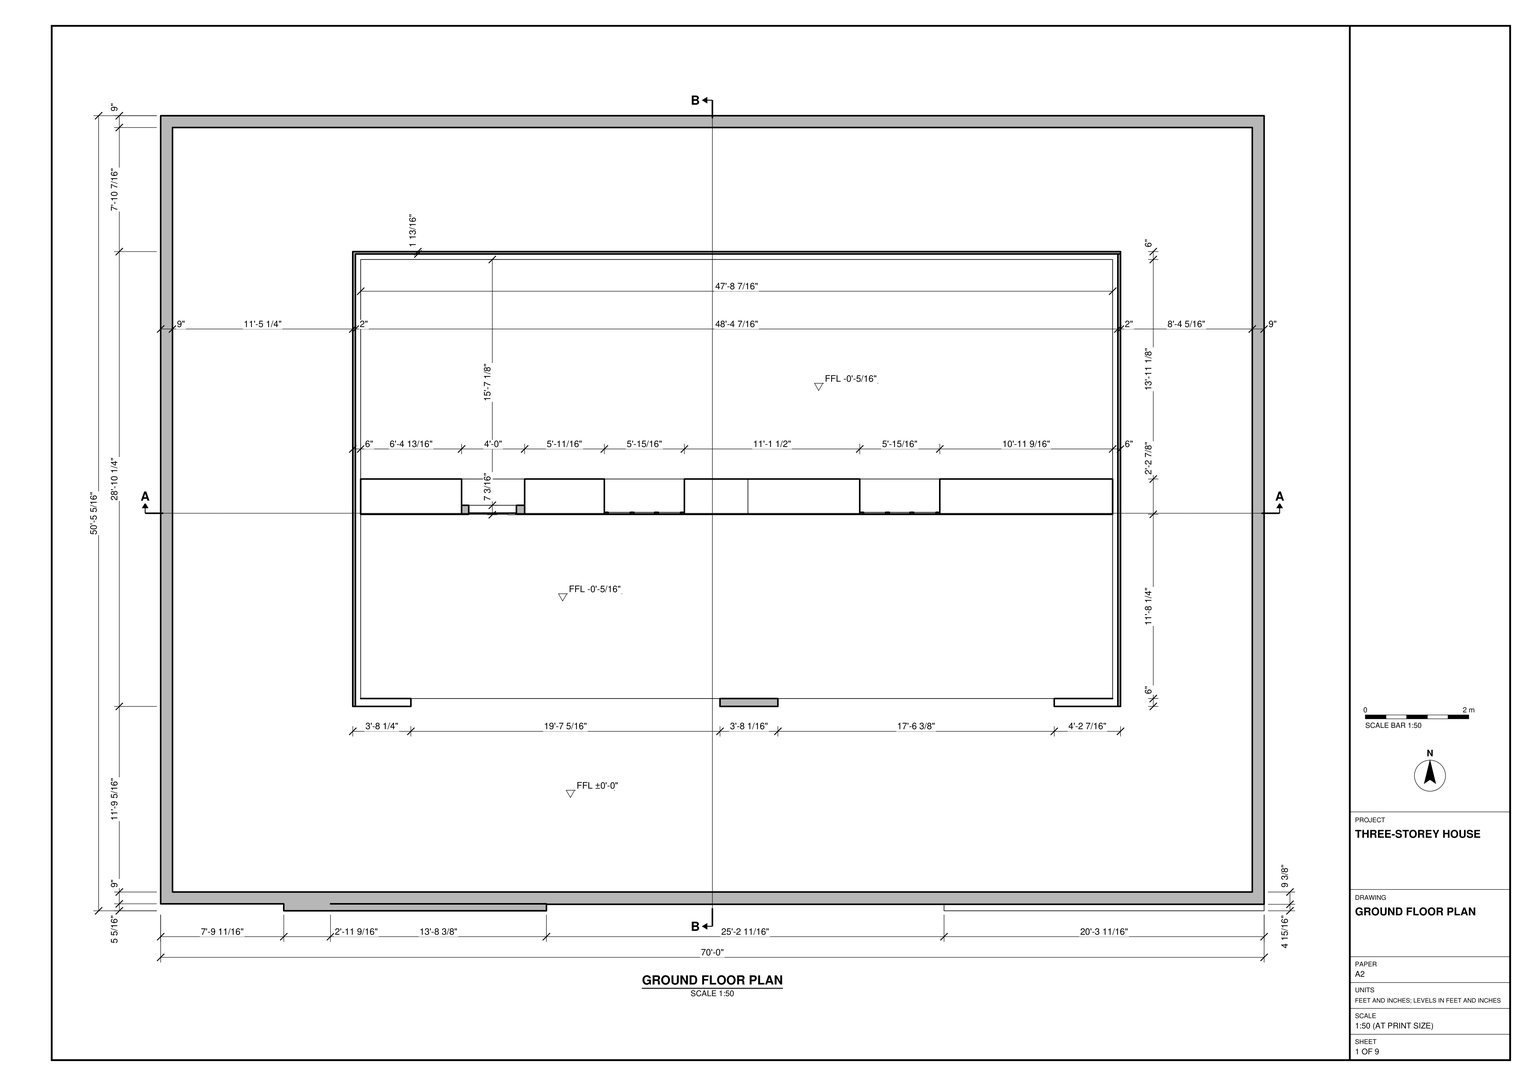
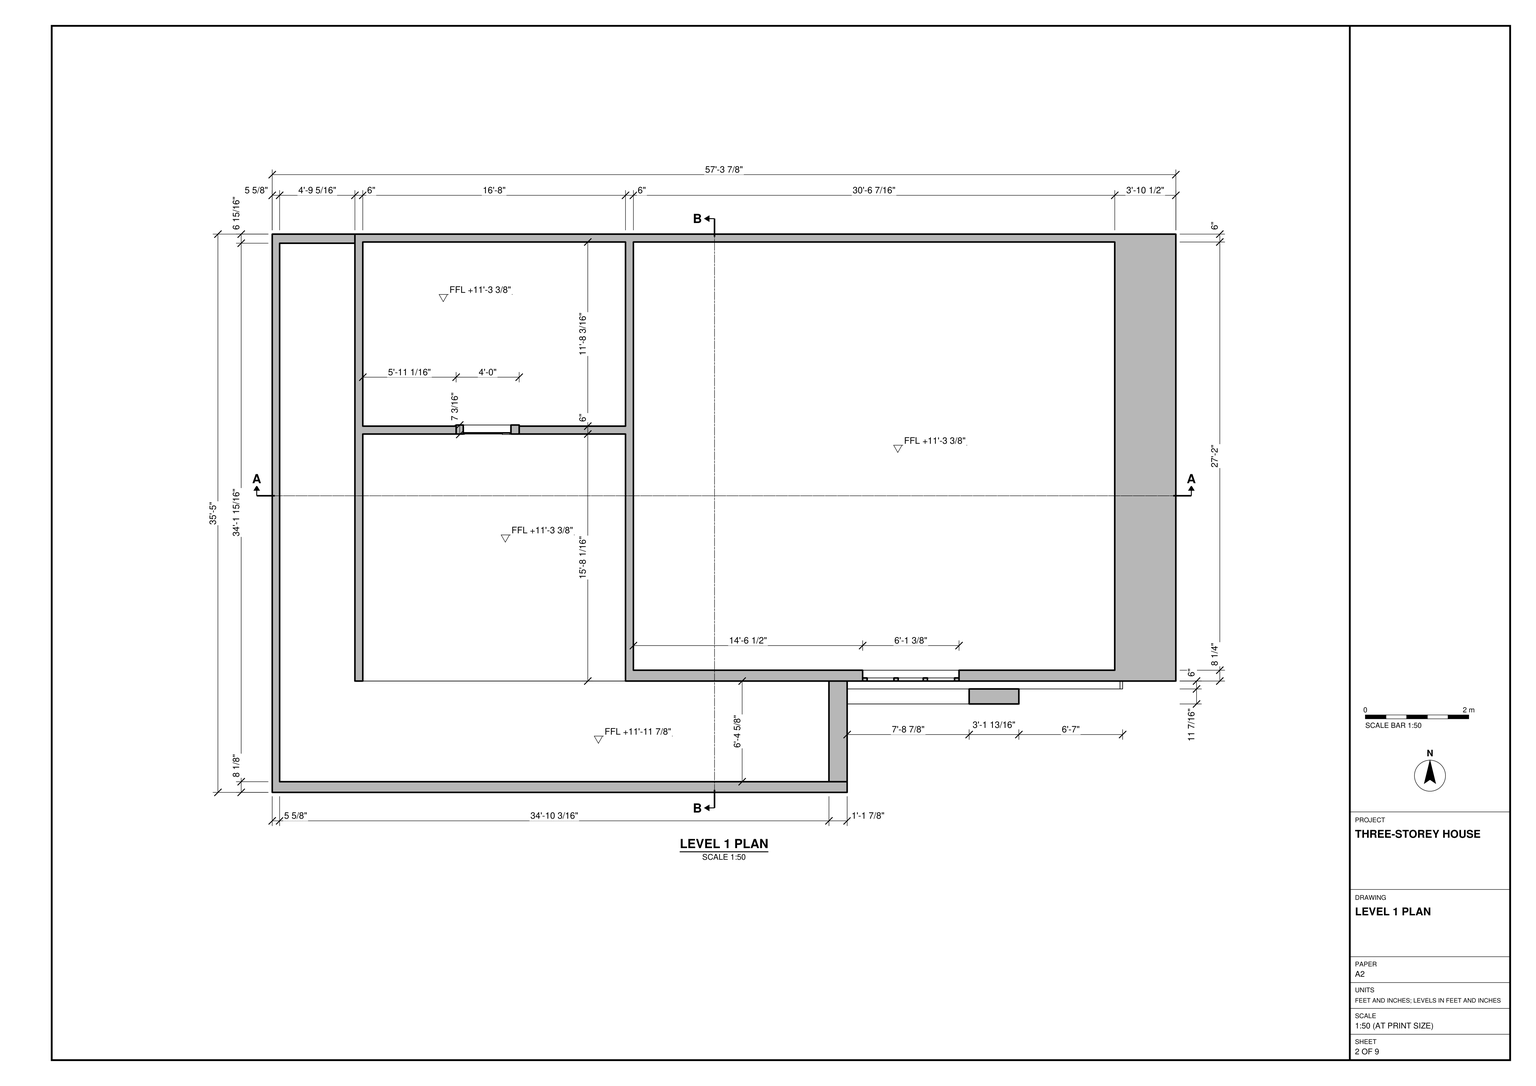
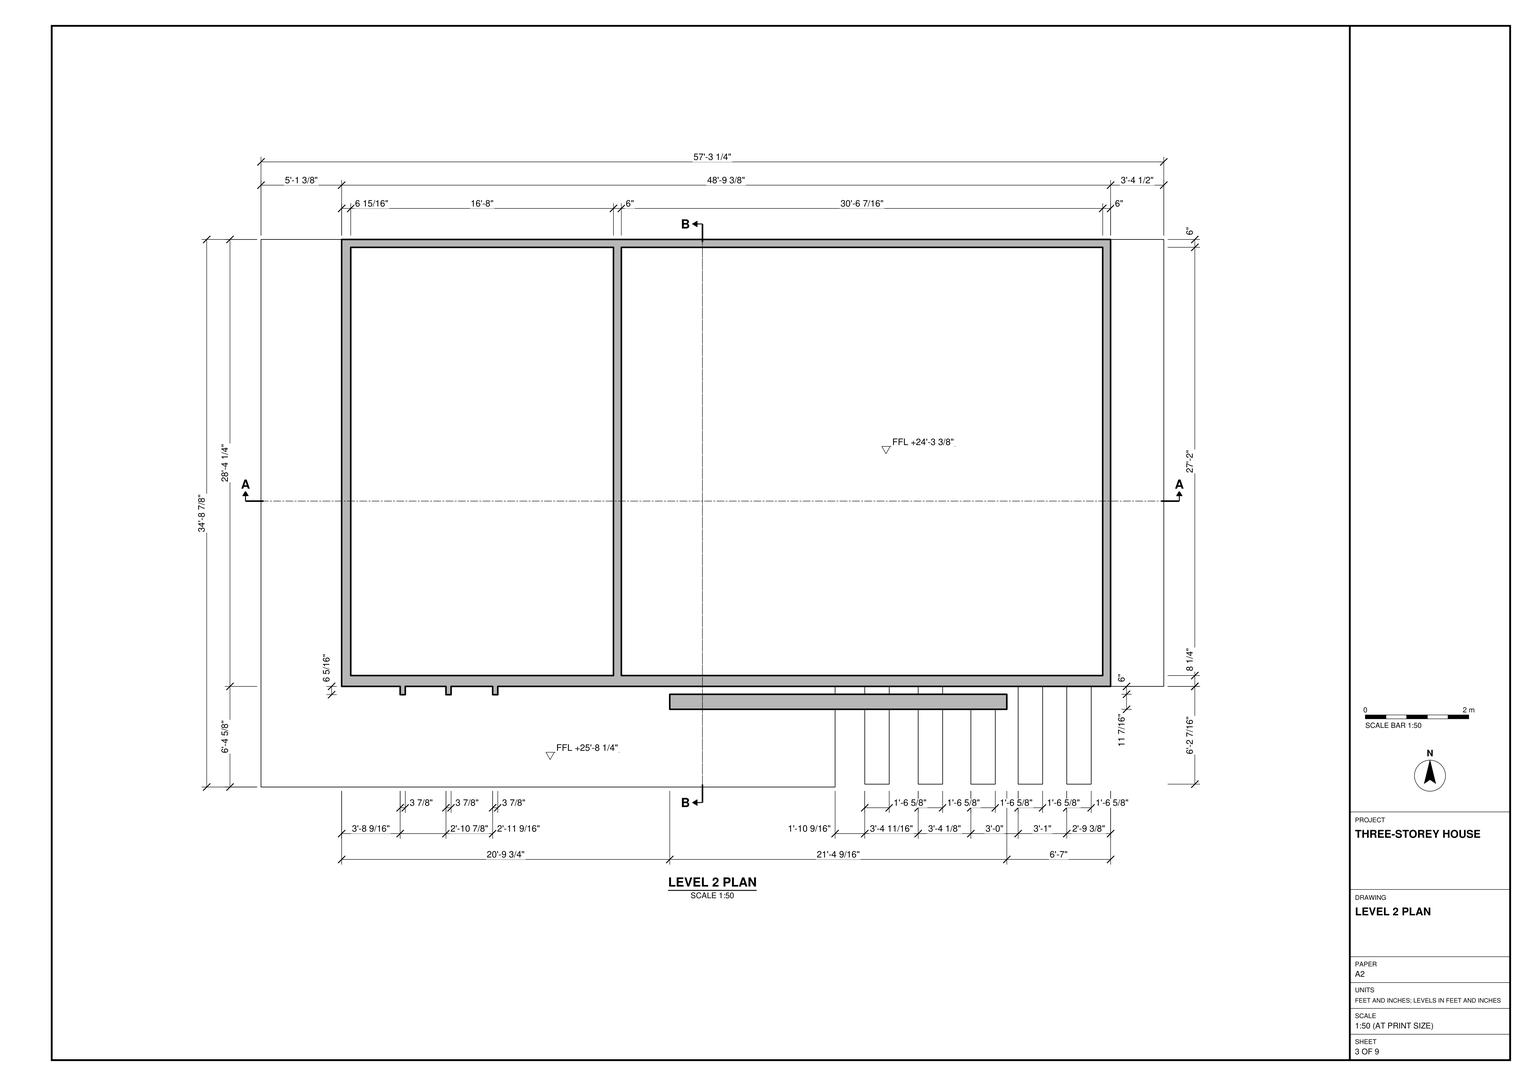
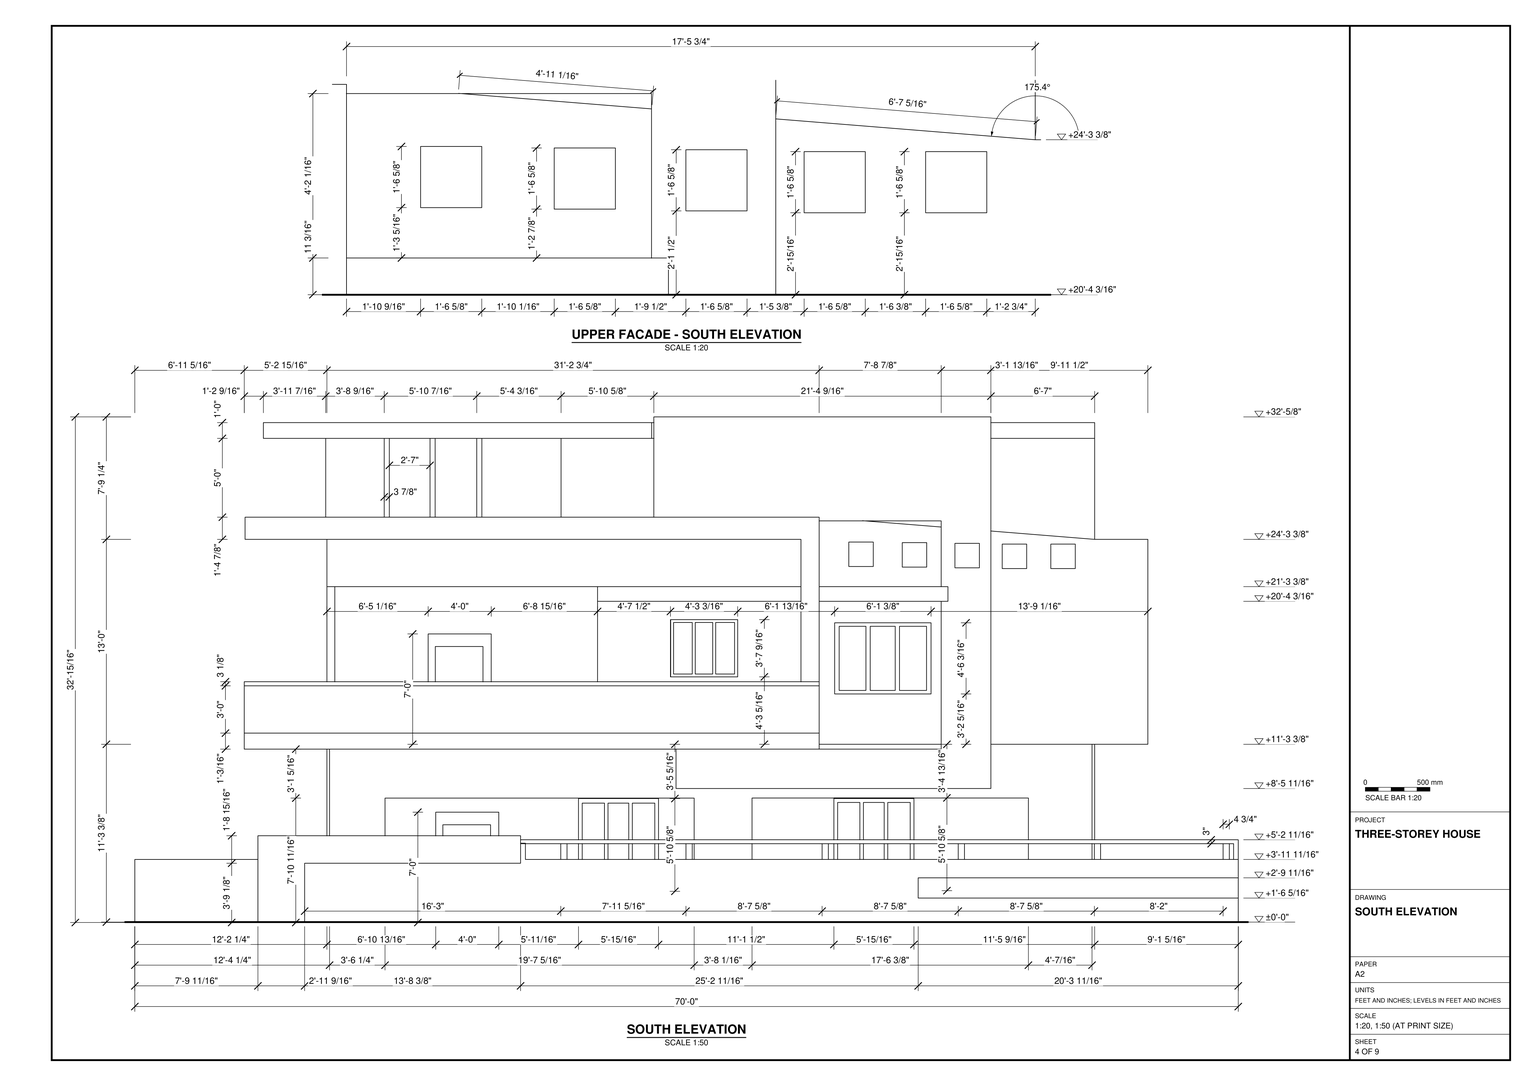
Build the house and its rectangular site perimeter in SketchUp using task_files/diagram_01.pdf. Work in feet and inches. The overall model is 70'-0" along X, 50'-5 5/16" along Y and 32'-15/16" high. Set the ground datum at ±0'-0", Level 1 at +11'-3 3/8" and Level 2 at +24'-3 3/8".

Set out the ground-floor footprint inside the perimeter, preserving the different setbacks on each side. Form the two wide openings along the front edge and the wall with openings between the front and rear spaces. At Level 1, lay out the smaller spaces on the left and the larger space on the right. Follow the stepped slab edge around the left side and across the front-left portion. At Level 2, align the lengthwise dividing wall with the division below. Model the roof edges, parallel projections at the front right and the member running across them.

Use the wall and slab thicknesses shown, and place door and window openings in the corresponding wall bays. Include stairs, built-in joinery and main furniture where shown. Keep shell elements such as walls, slabs and roof, and each furniture or joinery piece, in separate groups or components. Use components for repeated parts. Decor and loose items may be any suitable library components. Save one SketchUp model as output_files/three_storey_house_stepped_slabs_and_projecting_beams.skp.

# SketchUp Ruby script. Lengths in inches.
U = 1.inch
M = Sketchup.active_model
def pt(a) = Geom::Point3d.new(a.map { |v| v * U })
def face(e, loops, mat)
  f = e.add_face(loops[0].map { |a| pt(a) })
  loops[1..].each { |l| e.add_face(l.map { |a| pt(a) }).erase! }
  f.material = f.back_material = mat if mat
  f
end
# faces: each face lists its corners as indices into pts; further lists are holes
def faces(e, pts, list, mat = nil) = list.each { |f| face(e, (f[0].is_a?(Array) ? f : [f]).map { |l| l.map { |i| pts[i] } }, mat) }
# xy, xz, yz: faces in a plane at the given z, y or x. An outline is a flat list of corners, or four numbers for a rectangle; further outlines are holes
def ring(l) = l.size == 4 ? [[l[0], l[1]], [l[2], l[1]], [l[2], l[3]], [l[0], l[3]]] : l.each_slice(2).to_a
def flat(e, list, mat, &to3) = list.each { |f| face(e, (f[0].is_a?(Array) ? f : [f]).map { |l| ring(l).map { |u, v| to3.(u, v) } }, mat) }
def xy(e, z, list, mat = nil) = flat(e, list, mat) { |x, y| [x, y, z] }
def xz(e, y, list, mat = nil) = flat(e, list, mat) { |x, z| [x, y, z] }
def yz(e, x, list, mat = nil) = flat(e, list, mat) { |y, z| [x, y, z] }
def lines(e, pts, list) = list.each { |a, b| e.add_line(pt(pts[a]), pt(pts[b])) }
# prism: a flat outline (further loops are holes) pulled along v
def prism(e, loops, v, mat = nil)
  f = face(e, loops, mat); d = Geom::Vector3d.new(v.map { |x| x * U })
  f.pushpull(f.normal.samedirection?(d) ? d.length : -d.length)
end
def box(e, o, s, mat = nil) = prism(e, [[o, [o[0] + s[0], o[1], o[2]], [o[0] + s[0], o[1] + s[1], o[2]], [o[0], o[1] + s[1], o[2]]]], [0, 0, s[2]], mat)
def at(x, y, z, deg = 0) = Geom::Transformation.translation(pt([x, y, z])) * Geom::Transformation.rotation(ORIGIN, Z_AXIS, deg.degrees)
def axes(o, x, y, z) = Geom::Transformation.new([*x, 0, *y, 0, *z, 0, *pt(o).to_a, 1])
def part(name) = M.definitions.add(name)
# library, detail: a bought-in or finely detailed component or shape, given as its bounding box
def library(name, o, s) = part(name).tap { |d| box(d.entities, o, s) }
def detail(e, o, s) = box(e.add_group.entities, o, s)
def put(e, d, t, mat = nil) = e.add_instance(d, t).tap { |i| i.material = mat if mat }
def group(e, t, mat = nil) = e.add_group.tap { |g| g.transformation = t; g.material = mat if mat }.entities
root = M.entities
M.materials.add("[0129_WhiteSmoke]").color = [245, 245, 245]
M.materials.add("[Color A08]").color = [102, 0, 0]
M.materials.add("[Color C08]").color = [86, 24, 0]
M.materials.add("[Color D02]").color = [255, 229, 153]
M.materials.add("[Color M00]").color = [255, 255, 255]
M.materials.add("[Granite Light Gray]").color = [149, 148, 144]
M.materials.add("[Metal Seamed]").color = [118, 119, 115]
M.materials.add("[Steel Brushed Stainless]").color = [183, 187, 190]
M.materials.add("[Stone Vein Gray]").color = [166, 165, 165]
M.materials.add("[Translucent Glass Gray]").color = [128, 128, 128]
M.materials["[Translucent Glass Gray]"].alpha = 0.5
M.materials.add("[Wood Veneer 01]").color = [120, 70, 37]
c1 = part("Group\#1")
xy(c1.entities,0,[[0,0,83.9375,6]],"[Color C08]")
xy(c1.entities,3.92,[[3.92,0,27.24,6],[30.96,0,52.74,6],[56.46,0,80.02,6]])
xy(c1.entities,75.45,[[3.92,0,27.24,6],[30.96,0,52.74,6],[56.46,0,80.02,6]],"[Color C08]")
xy(c1.entities,79.375,[[0,0,83.9375,6]],"[Color C08]")
xz(c1.entities,0,[[[0,0,83.9375,79.375],[56.46,3.92,80.02,75.45],[3.92,3.92,27.24,75.45],[30.96,3.92,52.74,75.45]]],"[Color C08]")
xz(c1.entities,0,[[3.92,3.92,27.24,75.45],[30.96,3.92,52.74,75.45],[56.46,3.92,80.02,75.45]],"[Translucent Glass Gray]")
xz(c1.entities,6,[[[0,0,83.9375,79.375],[3.92,3.92,80.02,75.45]],[27.24,3.92,30.96,75.45],[52.74,3.92,56.46,75.45]],"[Color C08]")
yz(c1.entities,0,[[0,0,6,79.375]],"[Color C08]")
yz(c1.entities,3.92,[[0,3.92,6,75.45]],"[Color C08]")
yz(c1.entities,27.24,[[0,3.92,6,75.45]],"[Color C08]")
yz(c1.entities,30.96,[[0,3.92,6,75.45]],"[Color C08]")
yz(c1.entities,52.74,[[0,3.92,6,75.45]],"[Color C08]")
yz(c1.entities,56.46,[[0,3.92,6,75.45]],"[Color C08]")
yz(c1.entities,80.02,[[0,3.92,6,75.45]],"[Color C08]")
yz(c1.entities,83.9375,[[0,0,6,79.375]],"[Color C08]")
c2 = part("Group\#2")
xy(c2.entities,0,[[0,0.3125,48,7.1875]])
xy(c2.entities,2.93,[[5.43,0.3125,41.74,1.1875]])
xy(c2.entities,2.93,[[5.43,1.1875,41.74,7.1875]],"[Wood Veneer 01]")
xy(c2.entities,74.42,[[5.43,0.3125,41.74,1.1875]])
xy(c2.entities,74.42,[[5.43,1.1875,41.74,7.1875]],"[Wood Veneer 01]")
xy(c2.entities,84,[[0,0.3125,48,7.1875]],"[Wood Veneer 01]")
xz(c2.entities,0,[[38.04,38.52,38.8,38.62,39.51,38.91,40.12,39.38,40.59,39.99,40.88,40.69,40.98,41.46,40.88,42.22,40.59,42.92,40.12,43.53,39.51,44,38.8,44.29,38.04,44.39,37.28,44.29,36.57,44,35.97,43.53,35.5,42.92,35.21,42.22,35.11,41.46,35.21,40.69,35.5,39.99,35.97,39.38,36.57,38.91,37.28,38.62]],"[Steel Brushed Stainless]")
xz(c2.entities,0.3125,[[[0,0,48,84],[5.43,2.93,41.74,74.42]]],"[Wood Veneer 01]")
xz(c2.entities,1.1875,[[[5.43,2.93,41.74,74.42],[38.04,38.52,37.28,38.62,36.57,38.91,35.97,39.38,35.5,39.99,35.21,40.69,35.11,41.46,35.21,42.22,35.5,42.92,35.97,43.53,36.57,44,37.28,44.29,38.04,44.39,38.8,44.29,39.51,44,40.12,43.53,40.59,42.92,40.88,42.22,40.98,41.46,40.88,40.69,40.59,39.99,40.12,39.38,39.51,38.91,38.8,38.62]]],"[Wood Veneer 01]")
xz(c2.entities,7.1875,[[[0,0,48,84],[5.43,2.93,41.74,74.42]]],"[Wood Veneer 01]")
yz(c2.entities,0,[[0.3125,0,7.1875,84]],"[Wood Veneer 01]")
yz(c2.entities,5.43,[[0.3125,2.93,1.1875,74.42]])
yz(c2.entities,5.43,[[1.1875,2.93,7.1875,74.42]],"[Wood Veneer 01]")
yz(c2.entities,41.74,[[0.3125,2.93,1.1875,74.42]])
yz(c2.entities,41.74,[[1.1875,2.93,7.1875,74.42]],"[Wood Veneer 01]")
yz(c2.entities,48,[[0.3125,0,7.1875,84]],"[Wood Veneer 01]")
p = [[37.28,1.1875,38.62],[38.04,1.1875,38.52],[38.04,0,38.52],[37.28,0,38.62],[38.8,1.1875,38.62],[38.8,0,38.62],
  [36.57,1.1875,38.91],[36.57,0,38.91],[39.51,1.1875,38.91],[39.51,0,38.91],[35.97,1.1875,39.38],[35.97,0,39.38],
  [40.12,1.1875,39.38],[40.12,0,39.38],[35.5,1.1875,39.99],[35.5,0,39.99],[40.59,1.1875,39.99],[40.59,0,39.99],
  [35.21,1.1875,40.69],[35.21,0,40.69],[40.88,1.1875,40.69],[40.88,0,40.69],[35.11,1.1875,41.46],[35.11,0,41.46],
  [40.98,1.1875,41.46],[40.98,0,41.46],[35.21,1.1875,42.22],[35.21,0,42.22],[40.88,1.1875,42.22],[40.88,0,42.22],
  [35.5,1.1875,42.92],[35.5,0,42.92],[40.59,1.1875,42.92],[40.59,0,42.92],[35.97,1.1875,43.53],[35.97,0,43.53],
  [40.12,1.1875,43.53],[40.12,0,43.53],[36.57,1.1875,44],[36.57,0,44],[39.51,1.1875,44],[39.51,0,44],
  [37.28,1.1875,44.29],[37.28,0,44.29],[38.8,1.1875,44.29],[38.8,0,44.29],[38.04,1.1875,44.39],[38.04,0,44.39]]
faces(c2.entities,p,[[0,1,2,3],[1,4,5,2],[6,0,3,7],[4,8,9,5],[10,6,7,11],[8,12,13,9],[14,10,11,15],[12,16,17,13],
  [18,14,15,19],[16,20,21,17],[22,18,19,23],[20,24,25,21],[26,22,23,27],[24,28,29,25],[30,26,27,31],[28,32,33,29],
  [34,30,31,35],[32,36,37,33],[38,34,35,39],[36,40,41,37],[42,38,39,43],[40,44,45,41],[46,42,43,47],[44,46,47,45]],"[Steel Brushed Stainless]")
xy(root,0,[[[93.72,0,93.72,5.3125,0,5.3125,0,605.3125,840,605.3125,840,4.97,129.28,4.97,129.28,0],[9,14.3125,831,596.3125]],[146.24,155.6,148.24,501.85],[148.24,155.6,148.24,500.04,728.68,500.04,728.68,155.6,680.24,155.6,680.24,161.6,724.68,161.6,724.68,495.85,152.24,495.85,152.24,161.6,190.48,161.6,190.48,155.6],[425.8,155.6,469.85,161.6],[728.68,155.6,730.68,500.04],
  [152.24,161.6,724.68,161.6,724.68,301.85,277.07,301.85,277.07,328.73,229.07,328.73,229.07,301.85,152.24,301.85],[152.24,301.85,229.07,328.73],[277.07,301.85,447.06,328.73],[447.06,301.85,724.68,328.73],[152.24,328.73,724.68,495.85],
  [148.24,500.04,730.68,501.85]])
xy(root,0.3125,[[[9,14.3125,831,596.3125],[146.24,155.6,146.24,501.85,730.68,501.85,730.68,155.6,680.24,155.6,680.24,161.6,469.85,161.6,469.85,155.6,425.8,155.6,425.8,161.6,190.48,161.6,190.48,155.6]]])
xy(root,18.6,[[596.34,0,840,4.97]],"[Granite Light Gray]")
xy(root,23.75,[[337.74,301.85,398.68,328.73]])
xy(root,24.25,[[532.18,301.85,593.11,328.73]])
xy(root,34.02,[[596.34,0,840,4.97]],"[Granite Light Gray]")
xy(root,45.12,[[129.28,4.97,293.65,5.3125]])
xy(root,45.12,[[129.28,0,293.65,4.97]],"[Granite Light Gray]")
xy(root,48,[[[297.35,4.97,836.45,14.3125],[326.64,7.73,326.03,7.82,325.45,8.05,324.96,8.43,324.58,8.92,324.35,9.5,324.27,10.11,324.35,10.72,324.58,11.3,324.96,11.79,325.45,12.17,326.03,12.4,326.64,12.48,327.26,12.4,327.83,12.17,328.32,11.79,328.7,11.3,328.93,10.72,329.02,10.11,328.93,9.5,328.7,8.92,328.32,8.43,327.83,8.05,327.26,7.82],[629.2,7.73,628.59,7.82,628.02,8.05,627.52,8.43,627.15,8.92,626.91,9.5,626.83,10.11,626.91,10.72,627.15,11.3,627.52,11.79,628.02,12.17,628.59,12.4,629.2,12.48,629.82,12.4,630.39,12.17,630.88,11.79,631.26,11.3,631.5,10.72,631.58,10.11,631.5,9.5,631.26,8.92,630.88,8.43,630.39,8.05,629.82,7.82],[525.58,7.73,524.96,7.82,524.39,8.05,523.9,8.43,523.52,8.92,523.28,9.5,523.2,10.11,523.28,10.72,523.52,11.3,523.9,11.79,524.39,12.17,524.96,12.4,525.58,12.48,526.19,12.4,526.77,12.17,527.26,11.79,527.64,11.3,527.87,10.72,527.95,10.11,527.87,9.5,527.64,8.92,527.26,8.43,526.77,8.05,526.19,7.82],[421.95,7.73,421.34,7.82,420.77,8.05,420.27,8.43,419.9,8.92,419.66,9.5,419.58,10.11,419.66,10.72,419.9,11.3,420.27,11.79,420.77,12.17,421.34,12.4,421.95,12.48,422.57,12.4,423.14,12.17,423.63,11.79,424.01,11.3,424.25,10.72,424.33,10.11,424.25,9.5,424.01,8.92,423.63,8.43,423.14,8.05,422.57,7.82],[830.83,7.73,830.21,7.82,829.64,8.05,829.15,8.43,828.77,8.92,828.53,9.5,828.45,10.11,828.53,10.72,828.77,11.3,829.15,11.79,829.64,12.17,830.21,12.4,830.83,12.48,831.44,12.4,832.02,12.17,832.51,11.79,832.89,11.3,833.12,10.72,833.2,10.11,833.12,9.5,832.89,8.92,832.51,8.43,832.02,8.05,831.44,7.82],[732.83,7.73,732.21,7.82,731.64,8.05,731.15,8.43,730.77,8.92,730.53,9.5,730.45,10.11,730.53,10.72,730.77,11.3,731.15,11.79,731.64,12.17,732.21,12.4,732.83,12.48,733.44,12.4,734.02,12.17,734.51,11.79,734.89,11.3,735.12,10.72,735.2,10.11,735.12,9.5,734.89,8.92,734.51,8.43,734.02,8.05,733.44,7.82]],[0,5.3125,293.65,5.3125,293.65,14.3125,9,14.3125,9,596.3125,831,596.3125,831,14.3125,840,14.3125,840,605.3125,0,605.3125]])
xy(root,60,[[293.65,4.97,293.65,14.3125,831.44,14.3125,831.44,12.4,830.83,12.48,830.21,12.4,829.64,12.17,829.15,11.79,828.77,11.3,828.53,10.72,828.45,10.11,828.53,9.5,828.77,8.92,829.15,8.43,829.64,8.05,830.21,7.82,830.83,7.73,831.44,7.82,831.44,4.97],[326.64,7.73,327.26,7.82,327.83,8.05,328.32,8.43,328.7,8.92,328.93,9.5,329.02,10.11,328.93,10.72,328.7,11.3,328.32,11.79,327.83,12.17,327.26,12.4,326.64,12.48,326.03,12.4,325.45,12.17,324.96,11.79,324.58,11.3,324.35,10.72,324.27,10.11,324.35,9.5,324.58,8.92,324.96,8.43,325.45,8.05,326.03,7.82],[421.95,7.73,422.57,7.82,423.14,8.05,423.63,8.43,424.01,8.92,424.25,9.5,424.33,10.11,424.25,10.72,424.01,11.3,423.63,11.79,423.14,12.17,422.57,12.4,421.95,12.48,421.34,12.4,420.77,12.17,420.27,11.79,419.9,11.3,419.66,10.72,419.58,10.11,419.66,9.5,419.9,8.92,420.27,8.43,420.77,8.05,421.34,7.82],[525.58,7.73,526.19,7.82,526.77,8.05,527.26,8.43,527.64,8.92,527.87,9.5,527.95,10.11,527.87,10.72,527.64,11.3,527.26,11.79,526.77,12.17,526.19,12.4,525.58,12.48,524.96,12.4,524.39,12.17,523.9,11.79,523.52,11.3,523.28,10.72,523.2,10.11,523.28,9.5,523.52,8.92,523.9,8.43,524.39,8.05,524.96,7.82],[629.2,7.73,629.82,7.82,630.39,8.05,630.88,8.43,631.26,8.92,631.5,9.5,631.58,10.11,631.5,10.72,631.26,11.3,630.88,11.79,630.39,12.17,629.82,12.4,629.2,12.48,628.59,12.4,628.02,12.17,627.52,11.79,627.15,11.3,626.91,10.72,626.83,10.11,626.91,9.5,627.15,8.92,627.52,8.43,628.02,8.05,628.59,7.82],
  [732.83,7.73,733.44,7.82,734.02,8.05,734.51,8.43,734.89,8.92,735.12,9.5,735.2,10.11,735.12,10.72,734.89,11.3,734.51,11.79,734.02,12.17,733.44,12.4,732.83,12.48,732.21,12.4,731.64,12.17,731.15,11.79,730.77,11.3,730.53,10.72,730.45,10.11,730.53,9.5,730.77,8.92,731.15,8.43,731.64,8.05,732.21,7.82],[830.83,7.73,830.21,7.82,829.64,8.05,829.15,8.43,828.77,8.92,828.53,9.5,828.45,10.11,828.53,10.72,828.77,11.3,829.15,11.79,829.64,12.17,830.21,12.4,830.83,12.48,831.44,12.4,831.44,7.82],[831.44,7.82,832.02,8.05,832.51,8.43,832.89,8.92,833.12,9.5,833.2,10.11,833.12,10.72,832.89,11.3,832.51,11.79,832.02,12.17,831.44,12.4]])
xy(root,60.03,[[831.44,4.97,836.45,14.3125]])
xy(root,60.375,[[293.65,4.97,297.35,14.3125]])
xy(root,63,[[293.65,4.97,840,14.3125]],"[Color A08]")
xy(root,66.0625,[[93.72,0,293.65,5.3125]],"[Granite Light Gray]")
xy(root,84,[[229.07,301.85,277.07,328.73]])
xy(root,94.38,[[337.74,301.85,398.68,328.73],[532.18,301.85,593.11,328.73]])
xy(root,94.71,[[190.48,155.6,425.8,161.6]])
xy(root,94.77,[[469.85,155.6,680.24,161.6]])
xy(root,102,[[412,144.16,651.68,155.6]])
xy(root,132,[[83.31,76.85,83.31,501.85,146.24,501.85,146.24,155.6,412,155.6,412,144.16,520.97,144.16,520.97,76.85],[412,144.16,520.97,155.6]])
xy(root,132,[[520.97,144.16,613.85,155.6]],"[Color C08]")
xy(root,133.8125,[[152.24,301.85,447.06,328.73],[447.06,301.85,724.68,328.73]])
xy(root,135.6875,[[146.24,155.6,148.24,232.63],[148.24,155.6,148.24,232.63,152.24,232.63,152.24,161.6,520.97,161.6,520.97,155.6],[520.97,155.6,728.68,161.6],[728.68,155.6,730.68,161.6],[[352.25,161.6,352.25,349.66,271.3,349.66,271.3,355.66,352.25,355.66,352.25,495.85,152.24,495.85,152.24,355.66,223.3,355.66,223.3,349.66,152.24,349.66,152.24,232.63,148.24,232.63,148.24,500.04,728.68,500.04,728.68,161.6],[358.25,169.85,724.68,495.85]],
  [152.24,161.6,352.25,161.6,352.25,349.66,271.3,349.66,271.3,355.66,223.3,355.66,223.3,349.66,152.24,349.66],[728.68,161.6,730.68,500.04],[358.25,169.85,724.68,495.85],[152.24,355.66,352.25,495.85],[730.68,500.04,771.18,501.85]])
xy(root,135.6875,[[730.68,161.6,771.18,500.04]],"[Stone Vein Gray]")
xy(root,144.1875,[[83.31,76.85,83.31,501.85,146.24,501.85,146.24,494.93,88.95,494.93,88.95,84.98,520.97,84.98,520.97,76.85],[88.95,84.98,507.11,84.98,507.11,161.6,146.24,161.6,146.24,494.93,88.95,494.93]])
xy(root,173.99,[[532.76,161.6,606.14,169.85]])
xy(root,180.1875,[[83.31,76.85,83.31,501.85,146.24,501.85,146.24,494.93,88.95,494.93,88.95,84.98,520.97,84.98,520.97,76.85]])
xy(root,183.3125,[[83.31,76.85,520.97,76.85,520.97,84.98,88.95,84.98,88.95,494.93,146.24,494.93,146.24,501.85,83.31,501.85]],"[Metal Seamed]")
xy(root,187,[[407.94,161.6,458.94,169.85]])
xy(root,219.6875,[[223.3,349.66,271.3,355.66]])
xy(root,228.18,[[532.76,161.6,606.14,169.85]])
xy(root,230.57,[[407.94,161.6,458.94,169.85]])
xy(root,244.51,[[352.25,136.1,501.3,161.6],[501.3,136.1,507.11,161.6],[520.97,136.1,520.97,161.6,618.99,161.6,618.99,155.6,613.85,155.6,613.85,145.91,618.99,145.91,618.99,136.1],[613.85,145.91,618.99,155.6]])
xy(root,255.6875,[[352.25,136.1,507.11,161.6],[520.97,136.1,618.99,161.6],[152.24,161.6,352.25,169.85],[152.24,169.85,352.25,349.66],[358.25,169.85,724.68,495.85],
  [152.24,349.66,352.25,355.66],[152.24,355.66,352.25,495.85]])
xy(root,269.45,[[660.31,87.16,678.93,161.6],[697.31,87.16,715.93,161.6]],"[Color D02]")
xy(root,270.03,[[624.31,87.16,642.93,144.16]],"[Color D02]")
xy(root,270.57,[[584.21,87.16,602.84,161.6]],"[Color D02]")
xy(root,271.02,[[543.53,87.16,562.15,161.6]],"[Color D02]")
xy(root,288.08,[[660.31,87.16,678.93,161.6],[697.31,87.16,715.93,161.6]],"[Color D02]")
xy(root,288.65,[[624.31,87.16,642.93,144.16]],"[Color D02]")
xy(root,289.19,[[584.21,87.16,602.84,161.6]],"[Color D02]")
xy(root,289.65,[[543.53,87.16,562.15,161.6]],"[Color D02]")
xy(root,291.6875,[[83.93,84.98,507.11,161.6],[83.93,161.6,146.24,501.85],[152.24,169.85,352.25,495.85],[358.25,169.85,724.68,495.85]])
xy(root,291.6875,[[730.68,161.6,771.18,501.85]],"[Stone Vein Gray]")
xy(root,305.76,[[395.1,144.16,613.85,155.6]],"[Color C08]")
xy(root,308.5625,[[83.93,84.98,520.97,84.98,520.97,161.6,264.1875,161.6,264.1875,155.29,260.29,155.29,260.29,161.6,228.625,161.6,228.625,155.29,224.73,155.29,224.73,161.6,193.75,161.6,193.75,155.29,189.86,155.29,189.86,161.6,145.32,161.6,145.32,501.85,83.93,501.85]])
xy(root,368.5625,[[97.87,139.54,97.87,161.6,189.86,161.6,189.86,155.29,193.75,155.29,193.75,161.6,224.73,161.6,224.73,155.29,228.625,155.29,228.625,161.6,260.29,161.6,260.29,155.29,264.1875,155.29,264.1875,161.6,730.68,161.6,730.68,158.6,393.47,158.6,393.47,139.54],[189.86,155.29,193.75,161.6],[224.73,155.29,228.625,161.6],[260.29,155.29,264.1875,161.6],[97.87,161.6,145.32,501.85],
  [[145.32,161.6,145.32,501.85,152.24,501.85,152.24,169.85,352.25,169.85,352.25,495.85,152.24,495.85,152.24,501.85,730.68,501.85,730.68,161.6],[358.25,169.85,724.68,495.85]],[152.24,169.85,352.25,495.85],[358.25,169.85,724.68,495.85]])
xy(root,380.5625,[[97.87,139.54,393.47,139.54,393.47,158.6,730.68,158.6,730.68,501.85,97.87,501.85]])
xy(root,384.9375,[[395.1,144.16,651.68,155.6]],"[Color C08]")
xz(root,0,[[93.72,0,129.28,0,129.28,45.12,293.65,45.12,293.65,66.0625,93.72,66.0625],[596.34,18.6,840,34.02]],"[Granite Light Gray]")
xz(root,4.97,[[129.28,0,840,0,840,18.6,596.34,18.6,596.34,34.02,840,34.02,840,48,297.35,48,297.35,60,293.65,60,293.65,45.12,129.28,45.12],[596.34,18.6,840,34.02],[293.65,60,297.35,60.375]])
xz(root,4.97,[[836.45,48,840,48,840,63,293.65,63,293.65,60.375,297.35,60.375,297.35,60,831.44,60,831.44,60.03,836.45,60.03]],"[Color A08]")
xz(root,5.3125,[[0,0,93.72,48],[129.28,45.12,293.65,48]])
xz(root,5.3125,[[93.72,48,293.65,66.0625]],"[Granite Light Gray]")
xz(root,14.3125,[[9,0,831,0.3125],[9,0.3125,9,48,293.65,48,293.65,60,297.35,60,297.35,48,831,48,831,0.3125],[836.45,48,836.45,60.03,831.44,60.03,831.44,60,297.35,60,297.35,60.375,293.65,60.375,293.65,63,840,63,840,48],[293.65,60,297.35,60.375]])
xz(root,76.85,[[83.31,132,520.97,144.1875]])
xz(root,76.85,[[83.31,180.1875,520.97,183.3125]],"[Metal Seamed]")
xz(root,76.85,[[83.31,144.1875,520.97,180.1875]],"[Translucent Glass Gray]")
xz(root,84.98,[[507.11,144.1875,520.97,180.1875],[507.11,180.1875,520.97,183.3125],[507.11,183.3125,520.97,183.3125,520.97,308.5625,83.93,308.5625,83.93,291.6875,507.11,291.6875]])
xz(root,84.98,[[88.95,180.1875,507.11,183.3125]],"[Metal Seamed]")
xz(root,84.98,[[88.95,144.1875,507.11,180.1875]],"[Translucent Glass Gray]")
xz(root,87.16,[[660.31,269.45,678.93,288.08],[697.31,269.45,715.93,288.08],[624.31,270.03,642.93,288.65],[584.21,270.57,602.84,289.19],[543.53,271.02,562.15,289.65]],"[Color D02]")
xz(root,136.1,[[352.25,244.51,507.11,255.6875],[520.97,244.51,618.99,255.6875]])
xz(root,139.54,[[97.87,368.5625,393.47,380.5625]])
xz(root,144.16,[[[412,102,651.68,102,651.68,384.9375,395.1,384.9375,395.1,305.76,613.85,305.76,613.85,132,412,132],[624.31,270.03,642.93,288.65]]],"[Color C08]")
xz(root,155.29,[[189.86,308.5625,193.75,368.5625],[224.73,308.5625,228.625,368.5625],[260.29,308.5625,264.1875,368.5625]])
xz(root,155.6,[[146.24,0,148.24,0.3125],[148.24,0,190.48,0.3125],[425.8,0,469.85,0.3125],[680.24,0,728.68,0.3125],[728.68,0,730.68,0.3125],
  [146.24,0.3125,148.24,132],[148.24,0.3125,190.48,0.3125,190.48,94.71,425.8,94.71,425.8,0.3125,469.85,0.3125,469.85,94.77,680.24,94.77,680.24,0.3125,728.68,0.3125,728.68,135.6875,651.68,135.6875,651.68,102,412,102,412,132,148.24,132],[728.68,0.3125,730.68,135.6875],[146.24,132,148.24,135.6875],[148.24,132,520.97,135.6875],
  [520.97,132,613.85,135.6875],[613.85,135.6875,613.85,305.76,395.1,305.76,395.1,384.9375,651.68,384.9375,651.68,135.6875]])
xz(root,158.6,[[393.47,368.5625,730.68,380.5625]])
xz(root,161.6,[[152.24,0,152.24,135.6875,724.68,135.6875,724.68,0,680.24,0,680.24,94.77,469.85,94.77,469.85,0,425.8,0,425.8,94.71,190.48,94.71,190.48,0],[190.48,0,425.8,0.3125],[469.85,0,680.24,0.3125],[152.24,135.6875,352.25,144.1875],[352.25,135.6875,352.25,144.1875,507.11,144.1875,507.11,255.6875,520.97,255.6875,520.97,135.6875],
  [146.24,144.1875,152.24,255.6875],[[352.25,144.1875,507.11,244.51],[407.94,187,458.94,230.57]],[501.3,244.51,507.11,255.6875],[520.97,244.51,618.99,255.6875],[507.11,255.6875,520.97,291.6875],
  [507.11,291.6875,520.97,303.6875],[507.11,303.6875,520.97,308.5625]])
xz(root,161.6,[[324.47,308.5625,397.05,368.5625]],"[0129_WhiteSmoke]")
xz(root,161.6,[[730.68,291.6875,730.68,368.5625,397.05,368.5625,397.05,308.5625,520.97,308.5625]],"[Color M00]")
xz(root,161.6,[[[520.97,135.6875,771.18,135.6875,771.18,291.6875,730.68,291.6875,520.97,308.5625,520.97,255.6875,618.99,255.6875,618.99,244.51,520.97,244.51],[532.76,173.99,606.14,228.18],[543.53,271.02,562.15,289.65],[584.21,270.57,602.84,289.19],[660.31,269.45,678.93,288.08],[697.31,269.45,715.93,288.08]],[146.24,255.6875,507.11,291.6875],[145.32,308.5625,189.86,368.5625],[193.75,308.5625,224.73,368.5625],[228.625,308.5625,260.29,368.5625],
  [264.1875,308.5625,324.47,368.5625]],"[Stone Vein Gray]")
xz(root,169.85,[[[358.25,135.6875,724.68,255.6875],[532.76,173.99,606.14,228.18],[407.94,187,458.94,230.57]],[152.24,255.6875,352.25,291.6875],[358.25,255.6875,724.68,291.6875],[152.24,291.6875,352.25,303.6875],[358.25,291.6875,724.68,368.5625],
  [152.24,303.6875,352.25,368.5625]])
xz(root,301.85,[[[152.24,0,229.07,0,229.07,84,277.07,84,277.07,0,724.68,0,724.68,133.8125,152.24,133.8125],[337.74,23.75,398.68,94.38],[532.18,24.25,593.11,94.38]]])
xz(root,328.73,[[[152.24,0,152.24,133.8125,447.06,133.8125,447.06,0,277.07,0,277.07,84,229.07,84,229.07,0],[337.74,23.75,398.68,94.38]],[[447.06,0,724.68,133.8125],[532.18,24.25,593.11,94.38]]])
xz(root,349.66,[[152.24,135.6875,223.3,135.6875,223.3,219.6875,271.3,219.6875,271.3,135.6875,352.25,135.6875,352.25,255.6875,152.24,255.6875]])
xz(root,355.66,[[152.24,135.6875,152.24,255.6875,352.25,255.6875,352.25,135.6875,271.3,135.6875,271.3,219.6875,223.3,219.6875,223.3,135.6875]])
xz(root,494.93,[[88.95,180.1875,146.24,183.3125]],"[Metal Seamed]")
xz(root,494.93,[[88.95,144.1875,146.24,180.1875]],"[Translucent Glass Gray]")
xz(root,495.85,[[152.24,135.6875,158.21,255.6875],[158.21,135.6875,182.9,255.6875],[182.9,135.6875,352.25,255.6875],[358.25,135.6875,724.68,255.6875],[152.24,255.6875,158.21,291.6875],
  [158.21,255.6875,182.9,291.6875],[182.9,255.6875,352.25,291.6875],[358.25,255.6875,419.28,291.6875],[419.28,255.6875,428.15,291.6875],[428.15,255.6875,724.68,291.6875],
  [152.24,291.6875,352.25,368.5625],[358.25,291.6875,724.68,368.5625]])
xz(root,500.04,[[148.24,0,728.68,135.6875],[728.68,0,730.68,135.6875]])
xz(root,501.85,[[146.24,0,148.24,0.3125],[148.24,0,730.68,0.3125],[146.24,0.3125,146.24,132,83.31,132,83.31,144.1875,146.24,144.1875,146.24,291.6875,83.93,291.6875,83.93,308.5625,145.32,308.5625,145.32,368.5625,730.68,368.5625,730.68,291.6875,771.18,291.6875,771.18,135.6875,730.68,135.6875,730.68,0.3125],[97.87,368.5625,730.68,380.5625]])
xz(root,501.85,[[83.31,180.1875,146.24,183.3125]],"[Metal Seamed]")
xz(root,501.85,[[83.31,144.1875,146.24,180.1875]],"[Translucent Glass Gray]")
xz(root,596.3125,[[9,0,831,0.3125],[9,0.3125,831,48]])
xz(root,605.3125,[[0,0,840,48]])
yz(root,0,[[5.3125,0,605.3125,48]])
yz(root,9,[[14.3125,0,596.3125,0.3125],[14.3125,0.3125,596.3125,48]])
yz(root,83.31,[[76.85,132,501.85,144.1875]])
yz(root,83.31,[[76.85,180.1875,501.85,183.3125]],"[Metal Seamed]")
yz(root,83.31,[[76.85,144.1875,501.85,180.1875]],"[Translucent Glass Gray]")
yz(root,83.93,[[84.98,291.6875,501.85,308.5625]])
yz(root,88.95,[[84.98,180.1875,494.93,183.3125]],"[Metal Seamed]")
yz(root,88.95,[[84.98,144.1875,494.93,180.1875]],"[Translucent Glass Gray]")
yz(root,93.72,[[0,0,5.3125,66.0625]],"[Granite Light Gray]")
yz(root,97.87,[[139.54,368.5625,501.85,380.5625]])
yz(root,129.28,[[0,0,4.97,45.12]],"[Granite Light Gray]")
yz(root,145.32,[[161.6,308.5625,501.85,368.5625]])
yz(root,146.24,[[155.6,0,501.85,0.3125],[155.6,0.3125,501.85,132],[155.6,132,232.63,135.6875],[161.6,144.1875,161.6,255.6875,501.85,255.6875,501.85,183.3125,494.93,183.3125,494.93,144.1875],[494.93,144.1875,501.85,180.1875],
  [494.93,180.1875,501.85,183.3125],[161.6,255.6875,501.85,291.6875]])
yz(root,148.24,[[155.6,0,500.04,135.6875]])
yz(root,152.24,[[301.85,0,328.73,133.8125],[161.6,135.6875,349.66,255.6875],[355.66,135.6875,495.85,255.6875],[169.85,255.6875,495.85,291.6875],[169.85,291.6875,495.85,303.6875],
  [169.85,303.6875,495.85,368.5625]])
yz(root,189.86,[[155.29,308.5625,161.6,368.5625]])
yz(root,190.48,[[155.6,0,161.6,0.3125],[155.6,0.3125,161.6,94.71]])
yz(root,193.75,[[155.29,308.5625,161.6,368.5625]])
yz(root,223.3,[[349.66,135.6875,355.66,219.6875]])
yz(root,224.73,[[155.29,308.5625,161.6,368.5625]])
yz(root,228.625,[[155.29,308.5625,161.6,368.5625]])
yz(root,229.07,[[301.85,0,328.73,84]])
yz(root,260.29,[[155.29,308.5625,161.6,368.5625]])
yz(root,264.1875,[[155.29,308.5625,161.6,368.5625]])
yz(root,271.3,[[349.66,135.6875,355.66,219.6875]])
yz(root,277.07,[[301.85,0,328.73,84]])
yz(root,293.65,[[4.97,45.12,5.3125,48],[4.97,48,5.3125,60],[5.3125,48,14.3125,60],[4.97,60,5.3125,60.375],[5.3125,60,14.3125,60.375],
  [4.97,60.375,5.3125,63],[5.3125,60.375,14.3125,63]])
yz(root,293.65,[[0,45.12,4.97,45.12,4.97,63,5.3125,63,5.3125,66.0625,0,66.0625]],"[Granite Light Gray]")
yz(root,297.35,[[4.97,48,14.3125,60.375]])
yz(root,337.74,[[301.85,23.75,328.73,94.38]])
yz(root,352.25,[[161.6,135.6875,161.6,244.51,136.1,244.51,136.1,255.6875,349.66,255.6875,349.66,135.6875],[355.66,135.6875,495.85,255.6875],[169.85,255.6875,495.85,291.6875],[169.85,291.6875,349.66,303.6875],[349.66,291.6875,495.85,368.5625],
  [169.85,303.6875,349.66,368.5625]])
yz(root,358.25,[[169.85,135.6875,495.85,255.6875],[169.85,255.6875,495.85,291.6875],[169.85,291.6875,495.85,368.5625]])
yz(root,393.47,[[139.54,368.5625,158.6,380.5625]])
yz(root,395.1,[[144.16,305.76,155.6,384.9375]],"[Color C08]")
yz(root,398.68,[[301.85,23.75,328.73,94.38]])
yz(root,407.94,[[161.6,187,169.85,230.57]])
yz(root,412,[[144.16,102,155.6,132]])
yz(root,425.8,[[155.6,0,161.6,0.3125],[155.6,0.3125,161.6,94.71]])
yz(root,458.94,[[161.6,187,169.85,230.57]])
yz(root,469.85,[[155.6,0,161.6,0.3125],[155.6,0.3125,161.6,94.77]])
yz(root,507.11,[[84.98,144.1875,84.98,291.6875,161.6,291.6875,161.6,255.6875,136.1,255.6875,136.1,244.51,161.6,244.51,161.6,144.1875],[136.1,244.51,161.6,255.6875]])
yz(root,520.97,[[76.85,132,155.6,132,155.6,135.6875,161.6,135.6875,161.6,244.51,136.1,244.51,136.1,255.6875,143.73,255.6875,143.73,308.5625,84.98,308.5625,84.98,144.1875,76.85,144.1875],[76.85,144.1875,84.98,180.1875],[76.85,180.1875,84.98,183.3125],[136.1,244.51,161.6,255.6875],[143.73,255.6875,161.6,308.5625]])
yz(root,532.18,[[301.85,24.25,328.73,94.38]])
yz(root,532.76,[[161.6,173.99,169.85,228.18]])
yz(root,543.53,[[87.16,271.02,161.6,289.65]],"[Color D02]")
yz(root,562.15,[[87.16,271.02,161.6,289.65]],"[Color D02]")
yz(root,584.21,[[87.16,270.57,161.6,289.19]],"[Color D02]")
yz(root,593.11,[[301.85,24.25,328.73,94.38]])
yz(root,596.34,[[0,18.6,4.97,34.02]],"[Granite Light Gray]")
yz(root,602.84,[[87.16,270.57,161.6,289.19]],"[Color D02]")
yz(root,606.14,[[161.6,173.99,169.85,228.18]])
yz(root,613.85,[[144.16,132,155.6,244.51],[144.16,244.51,155.6,305.76]],"[Color C08]")
yz(root,618.99,[[136.1,244.51,161.6,255.6875]])
yz(root,624.31,[[87.16,270.03,144.16,288.65]],"[Color D02]")
yz(root,642.93,[[87.16,270.03,144.16,288.65]],"[Color D02]")
yz(root,651.68,[[144.16,102,155.6,384.9375]],"[Color C08]")
yz(root,660.31,[[87.16,269.45,161.6,288.08]],"[Color D02]")
yz(root,678.93,[[87.16,269.45,161.6,288.08]],"[Color D02]")
yz(root,680.24,[[155.6,0,161.6,0.3125],[155.6,0.3125,161.6,94.77]])
yz(root,697.31,[[87.16,269.45,161.6,288.08]],"[Color D02]")
yz(root,715.93,[[87.16,269.45,161.6,288.08]],"[Color D02]")
yz(root,724.68,[[301.85,0,328.73,133.8125],[169.85,135.6875,495.85,255.6875],[169.85,255.6875,495.85,291.6875],[169.85,291.6875,495.85,368.5625]])
yz(root,728.68,[[155.6,0,500.04,135.6875]])
yz(root,730.68,[[155.6,0,500.04,0.3125],[500.04,0,501.85,0.3125],[155.6,0.3125,500.04,135.6875],[500.04,0.3125,501.85,135.6875],[161.6,291.6875,501.85,368.5625],
  [158.6,368.5625,161.6,380.5625],[161.6,368.5625,501.85,380.5625]])
yz(root,771.18,[[161.6,135.6875,501.85,291.6875]],"[Stone Vein Gray]")
yz(root,831,[[14.3125,0,596.3125,0.3125],[14.3125,0.3125,596.3125,48]])
yz(root,831.44,[[4.97,60,14.3125,60.03]])
yz(root,836.45,[[4.97,48,14.3125,60.03]],"[Color A08]")
yz(root,840,[[4.97,0,605.3125,0,605.3125,48,14.3125,48,14.3125,63,4.97,63]])
yz(root,840,[[0,18.6,4.97,34.02]],"[Granite Light Gray]")
p = [[326.03,7.82,48],[326.64,7.73,48],[326.64,7.73,60],[326.03,7.82,60],[327.26,7.82,48],[327.26,7.82,60],
  [421.34,7.82,48],[421.95,7.73,48],[421.95,7.73,60],[421.34,7.82,60],[422.57,7.82,48],[422.57,7.82,60],
  [524.96,7.82,48],[525.58,7.73,48],[525.58,7.73,60],[524.96,7.82,60],[526.19,7.82,48],[526.19,7.82,60],
  [628.59,7.82,48],[629.2,7.73,48],[629.2,7.73,60],[628.59,7.82,60],[629.82,7.82,48],[629.82,7.82,60],
  [732.21,7.82,48],[732.83,7.73,48],[732.83,7.73,60],[732.21,7.82,60],[733.44,7.82,48],[733.44,7.82,60],
  [830.21,7.82,48],[830.83,7.73,48],[830.83,7.73,60],[830.21,7.82,60],[831.44,7.82,48],[831.44,7.82,60],
  [325.45,8.05,48],[325.45,8.05,60],[327.83,8.05,48],[327.83,8.05,60],[420.77,8.05,48],[420.77,8.05,60],
  [423.14,8.05,48],[423.14,8.05,60],[524.39,8.05,48],[524.39,8.05,60],[526.77,8.05,48],[526.77,8.05,60],
  [628.02,8.05,48],[628.02,8.05,60],[630.39,8.05,48],[630.39,8.05,60],[731.64,8.05,48],[731.64,8.05,60],
  [734.02,8.05,48],[734.02,8.05,60],[829.64,8.05,48],[829.64,8.05,60],[832.02,8.05,48],[832.02,8.05,60],
  [324.96,8.43,48],[324.96,8.43,60],[328.32,8.43,48],[328.32,8.43,60],[420.27,8.43,48],[420.27,8.43,60],
  [423.63,8.43,48],[423.63,8.43,60],[523.9,8.43,48],[523.9,8.43,60],[527.26,8.43,48],[527.26,8.43,60],
  [627.52,8.43,48],[627.52,8.43,60],[630.88,8.43,48],[630.88,8.43,60],[731.15,8.43,48],[731.15,8.43,60],
  [734.51,8.43,48],[734.51,8.43,60],[829.15,8.43,48],[829.15,8.43,60],[832.51,8.43,48],[832.51,8.43,60],
  [324.58,8.92,48],[324.58,8.92,60],[328.7,8.92,48],[328.7,8.92,60],[419.9,8.92,48],[419.9,8.92,60],
  [424.01,8.92,48],[424.01,8.92,60],[523.52,8.92,48],[523.52,8.92,60],[527.64,8.92,48],[527.64,8.92,60],
  [627.15,8.92,48],[627.15,8.92,60],[631.26,8.92,48],[631.26,8.92,60],[730.77,8.92,48],[730.77,8.92,60],
  [734.89,8.92,48],[734.89,8.92,60],[828.77,8.92,48],[828.77,8.92,60],[832.89,8.92,48],[832.89,8.92,60],
  [324.35,9.5,48],[324.35,9.5,60],[328.93,9.5,48],[328.93,9.5,60],[419.66,9.5,48],[419.66,9.5,60],
  [424.25,9.5,48],[424.25,9.5,60],[523.28,9.5,48],[523.28,9.5,60],[527.87,9.5,48],[527.87,9.5,60],
  [626.91,9.5,48],[626.91,9.5,60],[631.5,9.5,48],[631.5,9.5,60],[730.53,9.5,48],[730.53,9.5,60],
  [735.12,9.5,48],[735.12,9.5,60],[828.53,9.5,48],[828.53,9.5,60],[833.12,9.5,48],[833.12,9.5,60],
  [324.27,10.11,48],[324.27,10.11,60],[329.02,10.11,48],[329.02,10.11,60],[419.58,10.11,48],[419.58,10.11,60],
  [424.33,10.11,48],[424.33,10.11,60],[523.2,10.11,48],[523.2,10.11,60],[527.95,10.11,48],[527.95,10.11,60],
  [626.83,10.11,48],[626.83,10.11,60],[631.58,10.11,48],[631.58,10.11,60],[730.45,10.11,48],[730.45,10.11,60],
  [735.2,10.11,48],[735.2,10.11,60],[828.45,10.11,48],[828.45,10.11,60],[833.2,10.11,48],[833.2,10.11,60],
  [324.35,10.72,48],[324.35,10.72,60],[328.93,10.72,48],[328.93,10.72,60],[419.66,10.72,48],[419.66,10.72,60],
  [424.25,10.72,48],[424.25,10.72,60],[523.28,10.72,48],[523.28,10.72,60],[527.87,10.72,48],[527.87,10.72,60],
  [626.91,10.72,48],[626.91,10.72,60],[631.5,10.72,48],[631.5,10.72,60],[730.53,10.72,48],[730.53,10.72,60],
  [735.12,10.72,48],[735.12,10.72,60],[828.53,10.72,48],[828.53,10.72,60],[833.12,10.72,48],[833.12,10.72,60],
  [324.58,11.3,48],[324.58,11.3,60],[328.7,11.3,48],[328.7,11.3,60],[419.9,11.3,48],[419.9,11.3,60],
  [424.01,11.3,48],[424.01,11.3,60],[523.52,11.3,48],[523.52,11.3,60],[527.64,11.3,48],[527.64,11.3,60],
  [627.15,11.3,48],[627.15,11.3,60],[631.26,11.3,48],[631.26,11.3,60],[730.77,11.3,48],[730.77,11.3,60],
  [734.89,11.3,48],[734.89,11.3,60],[828.77,11.3,48],[828.77,11.3,60],[832.89,11.3,48],[832.89,11.3,60],
  [324.96,11.79,48],[324.96,11.79,60],[328.32,11.79,48],[328.32,11.79,60],[420.27,11.79,48],[420.27,11.79,60],
  [423.63,11.79,48],[423.63,11.79,60],[523.9,11.79,48],[523.9,11.79,60],[527.26,11.79,48],[527.26,11.79,60],
  [627.52,11.79,48],[627.52,11.79,60],[630.88,11.79,48],[630.88,11.79,60],[731.15,11.79,48],[731.15,11.79,60],
  [734.51,11.79,48],[734.51,11.79,60],[829.15,11.79,48],[829.15,11.79,60],[832.51,11.79,48],[832.51,11.79,60],
  [325.45,12.17,48],[325.45,12.17,60],[327.83,12.17,48],[327.83,12.17,60],[420.77,12.17,48],[420.77,12.17,60],
  [423.14,12.17,48],[423.14,12.17,60],[524.39,12.17,48],[524.39,12.17,60],[526.77,12.17,48],[526.77,12.17,60],
  [628.02,12.17,48],[628.02,12.17,60],[630.39,12.17,48],[630.39,12.17,60],[731.64,12.17,48],[731.64,12.17,60],
  [734.02,12.17,48],[734.02,12.17,60],[829.64,12.17,48],[829.64,12.17,60],[832.02,12.17,48],[832.02,12.17,60],
  [326.03,12.4,48],[326.03,12.4,60],[327.26,12.4,48],[327.26,12.4,60],[421.34,12.4,48],[421.34,12.4,60],
  [422.57,12.4,48],[422.57,12.4,60],[524.96,12.4,48],[524.96,12.4,60],[526.19,12.4,48],[526.19,12.4,60],
  [628.59,12.4,48],[628.59,12.4,60],[629.82,12.4,48],[629.82,12.4,60],[732.21,12.4,48],[732.21,12.4,60],
  [733.44,12.4,48],[733.44,12.4,60],[830.21,12.4,48],[830.21,12.4,60],[831.44,12.4,48],[831.44,12.4,60],
  [326.64,12.48,48],[326.64,12.48,60],[421.95,12.48,48],[421.95,12.48,60],[525.58,12.48,48],[525.58,12.48,60],
  [629.2,12.48,48],[629.2,12.48,60],[732.83,12.48,48],[732.83,12.48,60],[830.83,12.48,48],[830.83,12.48,60],
  [724.68,495.85,0],[724.68,495.85,135.6875],[146.24,232.63,135.6875],[146.24,501.85,135.6875],[152.24,495.85,0],[152.24,495.85,135.6875],
  [148.24,500.04,135.6875],[148.24,501.85,135.6875],[352.25,349.66,291.6875],[358.25,349.66,291.6875],[520.97,161.6,291.6875],[520.97,169.85,291.6875],
  [152.24,495.85,291.6875],[152.24,501.85,291.6875],[146.24,501.85,291.6875],[507.11,161.6,303.6875],[507.11,84.98,303.6875],[146.24,161.6,303.6875],
  [352.25,349.66,368.5625],[352.25,349.66,380.5625],[352.25,169.85,368.5625],[352.25,169.85,380.5625],[152.24,169.85,368.5625],[152.24,169.85,380.5625],
  [152.24,495.85,368.5625],[152.24,495.85,380.5625],[145.32,161.6,368.5625],[145.32,161.6,380.5625],[162.18,495.85,368.5625],[162.18,495.85,380.5625],
  [358.25,169.85,368.5625],[358.25,169.85,380.5625],[382.45,495.85,368.5625],[382.45,495.85,380.5625],[724.68,495.85,368.5625],[724.68,495.85,380.5625],
  [724.68,169.85,368.5625],[724.68,169.85,380.5625]]
faces(root,p,[[0,1,2,3],[1,4,5,2],[6,7,8,9],[7,10,11,8],[12,13,14,15],[13,16,17,14],[18,19,20,21],[19,22,23,20],
  [24,25,26,27],[25,28,29,26],[30,31,32,33],[31,34,35,32],[36,0,3,37],[4,38,39,5],[40,6,9,41],[10,42,43,11],
  [44,12,15,45],[16,46,47,17],[48,18,21,49],[22,50,51,23],[52,24,27,53],[28,54,55,29],[56,30,33,57],[34,58,59,35],
  [60,36,37,61],[38,62,63,39],[64,40,41,65],[42,66,67,43],[68,44,45,69],[46,70,71,47],[72,48,49,73],[50,74,75,51],
  [76,52,53,77],[54,78,79,55],[80,56,57,81],[58,82,83,59],[84,60,61,85],[62,86,87,63],[88,64,65,89],[66,90,91,67],
  [92,68,69,93],[70,94,95,71],[96,72,73,97],[74,98,99,75],[100,76,77,101],[78,102,103,79],[104,80,81,105],[82,106,107,83],
  [108,84,85,109],[86,110,111,87],[112,88,89,113],[90,114,115,91],[116,92,93,117],[94,118,119,95],[120,96,97,121],[98,122,123,99],
  [124,100,101,125],[102,126,127,103],[128,104,105,129],[106,130,131,107],[132,108,109,133],[110,134,135,111],[136,112,113,137],[114,138,139,115],
  [140,116,117,141],[118,142,143,119],[144,120,121,145],[122,146,147,123],[148,124,125,149],[126,150,151,127],[152,128,129,153],[130,154,155,131],
  [156,132,133,157],[134,158,159,135],[160,136,137,161],[138,162,163,139],[164,140,141,165],[142,166,167,143],[168,144,145,169],[146,170,171,147],
  [172,148,149,173],[150,174,175,151],[176,152,153,177],[154,178,179,155],[180,156,157,181],[158,182,183,159],[184,160,161,185],[162,186,187,163],
  [188,164,165,189],[166,190,191,167],[192,168,169,193],[170,194,195,171],[196,172,173,197],[174,198,199,175],[200,176,177,201],[178,202,203,179],
  [204,180,181,205],[182,206,207,183],[208,184,185,209],[186,210,211,187],[212,188,189,213],[190,214,215,191],[216,192,193,217],[194,218,219,195],
  [220,196,197,221],[198,222,223,199],[224,200,201,225],[202,226,227,203],[228,204,205,229],[206,230,231,207],[232,208,209,233],[210,234,235,211],
  [236,212,213,237],[214,238,239,215],[240,216,217,241],[218,242,243,219],[244,220,221,245],[222,246,247,223],[248,224,225,249],[226,250,251,227],
  [252,228,229,253],[230,254,255,231],[256,232,233,257],[234,258,259,235],[260,236,237,261],[238,262,263,239],[264,240,241,265],[242,266,267,243],
  [268,244,245,269],[246,270,271,247],[272,248,249,273],[250,274,275,251],[276,252,253,277],[254,276,277,255],[278,256,257,279],[258,278,279,259],
  [280,260,261,281],[262,280,281,263],[282,264,265,283],[266,282,283,267],[284,268,269,285],[270,284,285,271],[286,272,273,287],[274,286,287,275]],"[Color A08]")
lines(root,p,[[288,289],[290,291],[292,293],[294,295],[296,297],[298,299],[300,301],[302,301],[303,304],[303,305],[306,307],[308,309],
  [310,311],[312,313],[314,315],[316,317],[318,319],[320,321],[322,323],[324,325]])
put(root,c1,axes([532.76,161.6,173.99],[0.87416,0,0],[0,0.39671,0],[0,0,0.68268]))
put(root,c1,axes([407.76,161.6,187],[0.60982,0,0],[0,0.25389,0],[0,0,0.54882]))
put(root,c1,axes([337.74,301.85,23.75],[0.72599,0,0],[0,0.25389,0],[0,0,0.88976]))
put(root,c1,axes([532.18,301.85,24.25],[0.72599,0,0],[0,0.25389,0],[0,0,0.88976]))
put(root,c2,at(229.07,301.54,0))
put(root,c2,at(223.3,349.35,135.6875))
